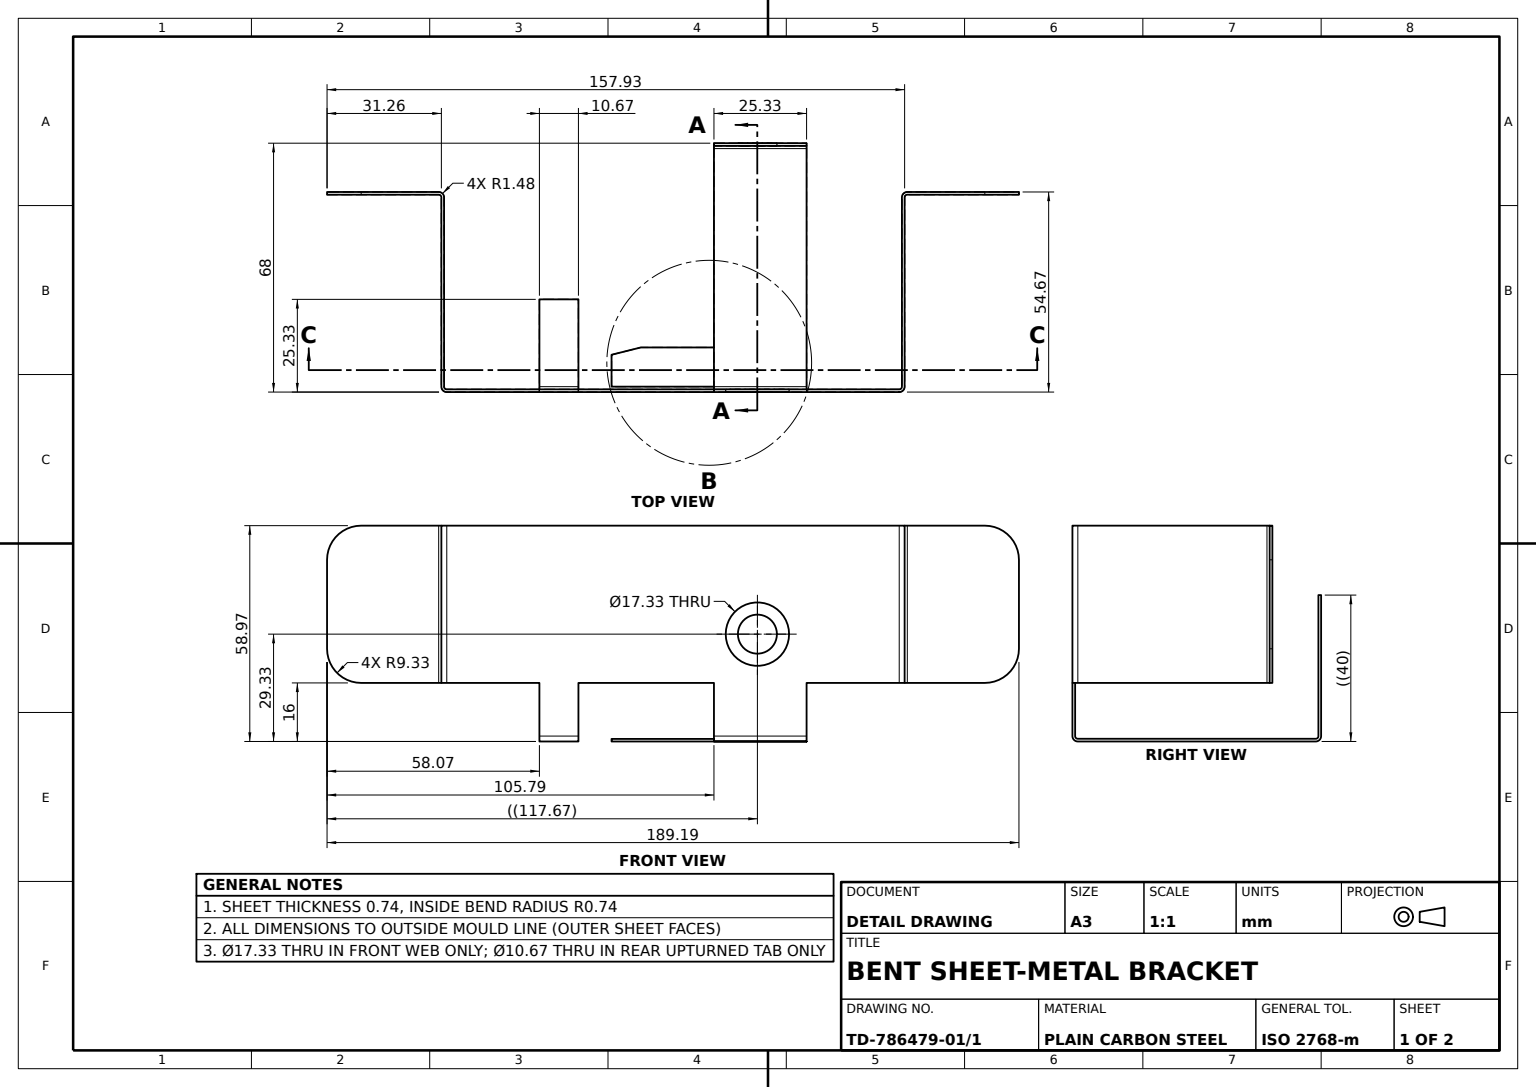
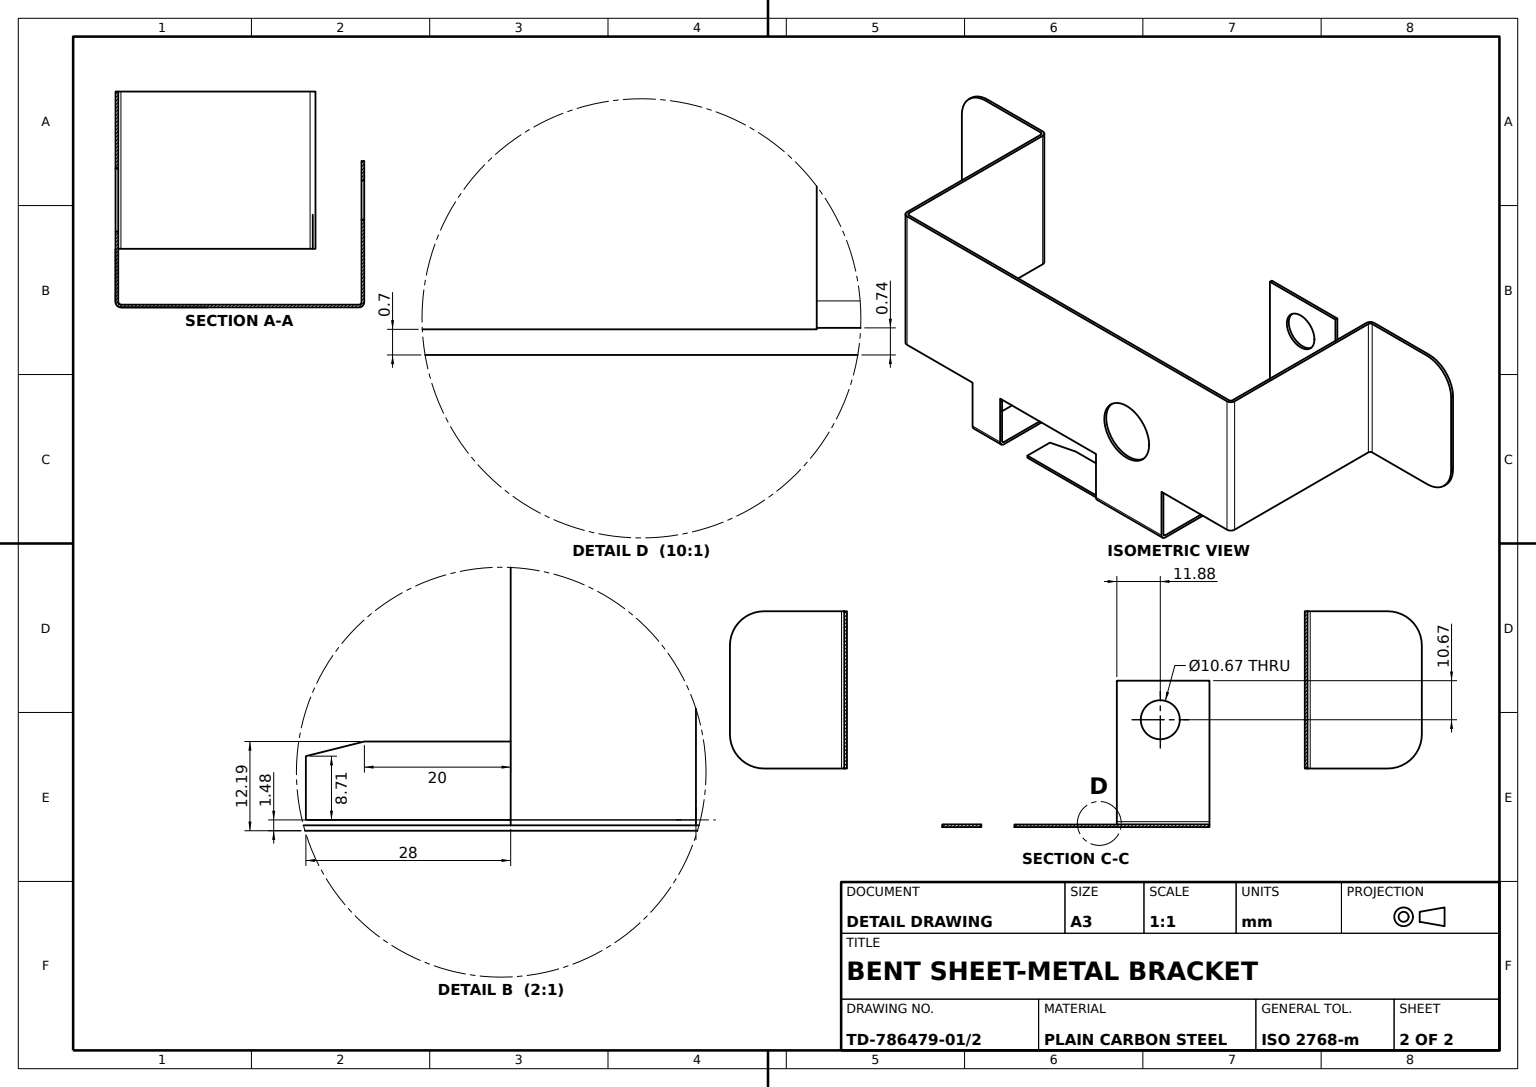
solid
v1 (11.1984,-36.745,-1.4766)
v2 (11.1984,-36.745,-66.5234)
e1 v1 v2 LINE
v3 (36.5284,-36.745,-1.4766)
e2 v3 v1 LINE
v4 (36.5284,-36.745,-66.5234)
e3 v4 v3 LINE
e4 v2 v4 LINE
face PLANE(AX(P(0,-36.745,0),D(0,1,0),D(0,0,1))) [-e1 -e2 -e3 -e4]
v5 (11.1984,-36.0084,0)
v6 (36.5284,-36.0084,0)
e5 v5 v6 LINE
v7 (11.1984,-37.485,-1.4766)
e6 v7 v5 CIRCLE(AX(P(11.1984,-36.0084,-1.4766),D(-1,0,0),D(0,0,1)),1.4766)
v8 (36.5284,-37.485,-1.4766)
e7 v7 v8 LINE
e8 v6 v8 CIRCLE(AX(P(36.5284,-36.0084,-1.4766),D(1,0,0),D(0,0,1)),1.4766)
face CYL(AX(P(11.1984,-36.0084,-1.4766),D(-1,0,0),D(0,-1,0)),1.4766) [-e5 -e6 e7 -e8]
v9 (-62.595,-21.485,-1.4766)
v10 (-63.335,-21.485,-1.4766)
e9 v9 v10 LINE
v11 (-61.8584,-21.485,-0.74)
e10 v11 v9 CIRCLE(AX(P(-61.8584,-21.485,-1.4766),D(0,-1,0),D(0,0,1)),0.7366)
v12 (-61.8584,-21.485,0)
e11 v11 v12 LINE
e12 v12 v10 CIRCLE(AX(P(-61.8584,-21.485,-1.4766),D(0,-1,0),D(0,0,1)),1.4766)
face PLANE(AX(P(-61.8584,-21.485,-1.4766),D(0,-1,0),D(0,0,-1))) [-e9 -e10 e11 e12]
v13 (-85.265,-21.485,-54.67)
v14 (-85.265,-21.485,-53.93)
e13 v13 v14 LINE
v15 (-94.595,-12.155,-53.93)
e14 v15 v14 CIRCLE(AX(P(-85.265,-12.155,-53.93),D(0,0,1),D(1,0,0)),9.33)
v16 (-94.595,-12.155,-54.67)
e15 v16 v15 LINE
e16 v16 v13 CIRCLE(AX(P(-85.265,-12.155,-54.67),D(0,0,1),D(1,0,0)),9.33)
face CYL(AX(P(-85.265,-12.155,-63.93),D(0,0,1),D(1,0,0)),9.33) [e13 -e14 -e15 e16]
v17 (85.265,-21.485,-54.67)
v18 (85.265,-21.485,-53.93)
e17 v17 v18 LINE
v19 (64.0716,-21.485,-53.93)
e18 v18 v19 LINE
v20 (64.0716,-21.485,-54.67)
e19 v19 v20 LINE
e20 v17 v20 LINE
face PLANE(AX(P(63.335,-21.485,-54.67),D(0,1,0),D(-1,0,0))) rev [e17 e18 e19 -e20]
v21 (11.1984,2.515,-68)
v22 (11.1984,2.515,-67.26)
e21 v21 v22 LINE
v23 (11.1984,-36.0084,-68)
e22 v23 v21 LINE
v24 (11.1984,-36.0084,-67.26)
e23 v24 v23 LINE
e24 v24 v22 LINE
face PLANE(AX(P(11.1984,2.515,-68),D(1,0,0),D(0,0,-1))) rev [-e21 -e22 -e23 e24]
v25 (-64.0716,-21.485,-54.67)
v26 (-64.0716,21.485,-54.67)
e25 v25 v26 LINE
v27 (-62.595,21.485,-53.1934)
e26 v27 v26 CIRCLE(AX(P(-64.0716,21.485,-53.1934),D(0,1,0),D(0,0,-1)),1.4766)
v28 (-62.595,-21.485,-53.1934)
e27 v28 v27 LINE
e28 v25 v28 CIRCLE(AX(P(-64.0716,-21.485,-53.1934),D(0,-1,0),D(0,0,-1)),1.4766)
face CYL(AX(P(-64.0716,-21.485,-53.1934),D(0,-1,0),D(0,0,-1)),1.4766) [e25 -e26 -e27 -e28]
v29 (36.5284,2.515,-67.26)
e29 v22 v29 LINE
v30 (36.5284,2.515,-68)
e30 v30 v29 LINE
e31 v21 v30 LINE
face PLANE(AX(P(36.5284,2.515,-68),D(0,-1,0),D(0,0,-1))) rev [e21 e29 -e30 -e31]
v31 (63.335,21.485,-53.1934)
v32 (62.595,21.485,-53.1934)
e32 v31 v32 LINE
v33 (62.595,21.485,-1.4766)
e33 v32 v33 LINE
v34 (63.335,21.485,-1.4766)
e34 v33 v34 LINE
e35 v31 v34 LINE
face PLANE(AX(P(63.335,21.485,-0.74),D(0,-1,0),D(1,0,0))) rev [e32 e33 e34 -e35]
v35 (-25.8584,-37.485,-25.33)
v36 (-25.8584,-36.745,-25.33)
e36 v35 v36 LINE
v37 (-25.8584,-36.745,-1.4766)
e37 v36 v37 LINE
v38 (-25.8584,-37.485,-1.4766)
e38 v37 v38 LINE
e39 v35 v38 LINE
face PLANE(AX(P(-25.8584,-37.485,-0.74),D(-1,0,0),D(0,0,1))) rev [e36 e37 e38 -e39]
v39 (-36.5284,-36.745,-25.33)
e40 v39 v36 LINE
v40 (-36.5284,-37.485,-25.33)
e41 v40 v35 LINE
e42 v40 v39 LINE
face PLANE(AX(P(-25.8584,-37.485,-25.33),D(0,0,1),D(0,-1,0))) rev [e40 -e36 -e41 e42]
v41 (36.5284,-21.485,0)
v42 (36.5284,-21.485,-0.74)
e43 v41 v42 LINE
e44 v6 v41 LINE
v43 (36.5284,-36.0084,-0.74)
e45 v43 v6 LINE
e46 v43 v42 LINE
face PLANE(AX(P(36.5284,-37.485,0),D(1,0,0),D(0,0,-1))) [-e43 -e44 -e45 e46]
v44 (-36.5284,-21.485,0)
e47 v12 v44 LINE
v45 (-36.5284,-36.0084,0)
e48 v45 v44 LINE
v46 (-25.8584,-36.0084,0)
e49 v45 v46 LINE
v47 (-25.8584,-21.485,0)
e50 v46 v47 LINE
v48 (11.1984,-21.485,0)
e51 v47 v48 LINE
e52 v5 v48 LINE
v49 (61.8584,-21.485,0)
e53 v41 v49 LINE
v50 (61.8584,21.485,0)
e54 v49 v50 LINE
v51 (-61.8584,21.485,0)
e55 v50 v51 LINE
e56 v51 v12 LINE
v52 (31.744549,-8.155,0)
v53 (14.414549,-8.155,0)
e57 v52 v53 CIRCLE(AX(P(23.079549,-8.155,0),D(0,0,-1),D(1,0,0)),8.665)
e58 v53 v52 CIRCLE(AX(P(23.079549,-8.155,0),D(0,0,-1),D(1,0,0)),8.665)
face PLANE(AX(P(36.5284,-37.485,0),D(0,0,-1),D(-1,0,0))) rev [e47 -e48 e49 e50 e51 -e52 e5 e44 e53 e54 e55 e56] [e57 e58]
v54 (61.8584,21.485,-0.74)
v55 (-61.8584,21.485,-0.74)
e59 v54 v55 LINE
e60 v55 v51 LINE
e61 v54 v50 LINE
face PLANE(AX(P(-63.335,21.485,-0.74),D(0,1,0),D(0,0,1))) [e59 e60 -e55 -e61]
e62 v25 v13 LINE
v56 (-64.0716,-21.485,-53.93)
e63 v56 v25 LINE
e64 v56 v14 LINE
face PLANE(AX(P(-94.595,-21.485,-54.67),D(0,1,0),D(0,0,1))) rev [-e62 -e63 e64 -e13]
e65 v3 v8 LINE
v57 (36.5284,-37.485,-66.5234)
e66 v57 v8 LINE
e67 v4 v57 LINE
face PLANE(AX(P(36.5284,-37.485,-0.74),D(-1,0,0),D(0,-1,0))) rev [e3 e65 -e66 -e67]
v58 (-36.5284,-21.485,-0.74)
e68 v58 v44 LINE
v59 (-36.5284,-36.0084,-0.74)
e69 v59 v58 LINE
e70 v59 v45 LINE
face PLANE(AX(P(-36.5284,-37.485,0),D(-1,0,0),D(0,0,1))) [e48 -e68 -e69 e70]
v60 (11.1984,-36.0084,-0.74)
e71 v60 v5 LINE
e72 v1 v60 CIRCLE(AX(P(11.1984,-36.0084,-1.4766),D(-1,0,0),D(0,0,1)),0.7366)
e73 v1 v7 LINE
face PLANE(AX(P(11.1984,-36.0084,-1.4766),D(1,0,0),D(0,0,-1))) rev [-e71 -e72 e73 e6]
v61 (94.595,12.155,-53.93)
v62 (94.595,-12.155,-53.93)
e74 v61 v62 LINE
v63 (94.595,-12.155,-54.67)
e75 v62 v63 LINE
v64 (94.595,12.155,-54.67)
e76 v64 v63 LINE
e77 v61 v64 LINE
face PLANE(AX(P(94.595,-21.485,-54.67),D(-1,0,0),D(0,-1,0))) rev [e74 e75 -e76 -e77]
e78 v63 v17 CIRCLE(AX(P(85.265,-12.155,-54.67),D(0,0,-1),D(1,0,0)),9.33)
v65 (64.0716,21.485,-54.67)
e79 v65 v20 LINE
v66 (85.265,21.485,-54.67)
e80 v65 v66 LINE
e81 v66 v64 CIRCLE(AX(P(85.265,12.155,-54.67),D(0,0,-1),D(1,0,0)),9.33)
face PLANE(AX(P(0,0,-54.67),D(0,0,1),D(1,0,0))) rev [e78 e20 -e79 e80 e81 e76]
v67 (-36.5284,-36.745,-1.4766)
e82 v37 v67 LINE
e83 v67 v59 CIRCLE(AX(P(-36.5284,-36.0084,-1.4766),D(-1,0,0),D(0,0,1)),0.7366)
v68 (-25.8584,-36.0084,-0.74)
e84 v59 v68 LINE
e85 v68 v37 CIRCLE(AX(P(-25.8584,-36.0084,-1.4766),D(1,0,0),D(0,0,1)),0.7366)
face CYL(AX(P(-36.5284,-36.0084,-1.4766),D(-1,0,0),D(0,-1,0)),0.7366) rev [e82 e83 e84 e85]
e86 v62 v18 CIRCLE(AX(P(85.265,-12.155,-53.93),D(0,0,-1),D(1,0,0)),9.33)
face CYL(AX(P(85.265,-12.155,-63.93),D(0,0,1),D(1,0,0)),9.33) [-e17 -e78 -e75 e86]
e87 v65 v32 CIRCLE(AX(P(64.0716,21.485,-53.1934),D(0,1,0),D(0,0,1)),1.4766)
v69 (62.595,-21.485,-53.1934)
e88 v69 v20 CIRCLE(AX(P(64.0716,-21.485,-53.1934),D(0,-1,0),D(0,0,1)),1.4766)
e89 v32 v69 LINE
face CYL(AX(P(64.0716,21.485,-53.1934),D(0,1,0),D(0,0,-1)),1.4766) [-e87 e79 -e88 -e89]
v70 (14.414549,-8.155,-0.74)
e90 v70 v53 LINE
v71 (31.744549,-8.155,-0.74)
e91 v71 v52 LINE
e92 v71 v70 CIRCLE(AX(P(23.079549,-8.155,-0.74),D(0,0,-1),D(1,0,0)),8.665)
face CYL(AX(P(23.079549,-8.155,-33.74),D(0,0,1),D(1,0,0)),8.665) rev [e90 -e57 -e91 e92]
v72 (62.595,-21.485,-1.4766)
e93 v72 v69 LINE
v73 (63.335,-21.485,-53.1934)
e94 v73 v69 LINE
v74 (63.335,-21.485,-1.4766)
e95 v74 v73 LINE
e96 v72 v74 LINE
face PLANE(AX(P(63.335,-21.485,-54.67),D(0,1,0),D(-1,0,0))) rev [e93 -e94 -e95 -e96]
v75 (61.8584,-21.485,-0.74)
e97 v75 v49 LINE
e98 v72 v75 CIRCLE(AX(P(61.8584,-21.485,-1.4766),D(0,-1,0),D(0,0,-1)),0.7366)
e99 v74 v49 CIRCLE(AX(P(61.8584,-21.485,-1.4766),D(0,-1,0),D(0,0,-1)),1.4766)
face PLANE(AX(P(61.8584,-21.485,-1.4766),D(0,1,0),D(0,0,1))) rev [-e97 -e98 e96 e99]
e100 v43 v3 CIRCLE(AX(P(36.5284,-36.0084,-1.4766),D(1,0,0),D(0,0,1)),0.7366)
face PLANE(AX(P(36.5284,-36.0084,-1.4766),D(1,0,0),D(0,0,-1))) [-e100 e45 e8 -e65]
v76 (17.744549,-8.155,-68)
v77 (17.744549,-8.155,-67.26)
e101 v76 v77 LINE
v78 (28.414549,-8.155,-68)
e102 v76 v78 CIRCLE(AX(P(23.079549,-8.155,-68),D(0,0,-1),D(0,-1,0)),5.335)
v79 (28.414549,-8.155,-67.26)
e103 v78 v79 LINE
e104 v77 v79 CIRCLE(AX(P(23.079549,-8.155,-67.26),D(0,0,-1),D(0,-1,0)),5.335)
face CYL(AX(P(23.079549,-8.155,-73.74),D(0,0,1),D(1,0,0)),5.335) rev [-e101 e102 e103 -e104]
v80 (64.0716,21.485,-53.93)
v81 (85.265,21.485,-53.93)
e105 v80 v81 LINE
e106 v66 v81 LINE
e107 v80 v65 LINE
face PLANE(AX(P(94.595,21.485,-54.67),D(0,-1,0),D(1,0,0))) rev [e105 -e106 -e80 -e107]
e108 v68 v46 LINE
e109 v46 v38 CIRCLE(AX(P(-25.8584,-36.0084,-1.4766),D(1,0,0),D(0,0,1)),1.4766)
face PLANE(AX(P(-25.8584,-36.0084,-1.4766),D(1,0,0),D(0,0,-1))) [-e38 -e85 e108 e109]
v82 (-85.265,21.485,-54.67)
v83 (-94.595,12.155,-54.67)
e110 v82 v83 CIRCLE(AX(P(-85.265,12.155,-54.67),D(0,0,1),D(1,0,0)),9.33)
e111 v82 v26 LINE
e112 v16 v83 LINE
face PLANE(AX(P(0,0,-54.67),D(0,0,1),D(1,0,0))) rev [-e110 e111 -e25 e62 -e16 e112]
v84 (-63.335,21.485,-1.4766)
e113 v84 v10 LINE
v85 (-63.335,21.485,-53.1934)
e114 v84 v85 LINE
v86 (-63.335,-21.485,-53.1934)
e115 v86 v85 LINE
e116 v86 v10 LINE
face PLANE(AX(P(-63.335,0,0),D(1,0,0),D(0,0,-1))) rev [-e113 e114 -e115 e116]
v87 (-94.595,12.155,-53.93)
e117 v15 v87 LINE
e118 v83 v87 LINE
face PLANE(AX(P(-94.595,21.485,-54.67),D(1,0,0),D(0,0,-1))) rev [e117 -e118 -e112 e15]
v88 (-8.8016,-36.785,-12.19)
v89 (11.1984,-36.785,-12.19)
e119 v88 v89 LINE
v90 (11.1984,-37.485,-12.19)
e120 v89 v90 LINE
v91 (-8.8016,-37.485,-12.19)
e121 v91 v90 LINE
e122 v88 v91 LINE
face PLANE(AX(P(11.1984,-36.785,-12.19),D(0,0,-1),D(0,1,0))) [e119 e120 -e121 -e122]
e123 v67 v39 LINE
face PLANE(AX(P(0,-36.745,0),D(0,1,0),D(0,0,1))) [-e37 -e40 -e123 -e82]
e124 v60 v43 LINE
face CYL(AX(P(11.1984,-36.0084,-1.4766),D(-1,0,0),D(0,-1,0)),0.7366) rev [e124 e100 e2 e72]
v92 (-62.595,21.485,-1.4766)
e125 v92 v27 LINE
e126 v9 v92 LINE
e127 v28 v9 LINE
face PLANE(AX(P(-62.595,0,0),D(1,0,0),D(0,0,-1))) [-e125 -e126 -e127 e27]
e128 v70 v71 CIRCLE(AX(P(23.079549,-8.155,-0.74),D(0,0,-1),D(1,0,0)),8.665)
face CYL(AX(P(23.079549,-8.155,-33.74),D(0,0,1),D(1,0,0)),8.665) rev [e91 -e58 -e90 e128]
e129 v92 v55 CIRCLE(AX(P(-61.8584,21.485,-1.4766),D(0,1,0),D(0,0,1)),0.7366)
e130 v55 v11 LINE
face CYL(AX(P(-61.8584,21.485,-1.4766),D(0,1,0),D(-1,0,0)),0.7366) rev [e129 e130 e10 e126]
v93 (-25.8584,-21.485,-0.74)
e131 v93 v47 LINE
e132 v68 v93 LINE
face PLANE(AX(P(-25.8584,-37.485,0),D(-1,0,0),D(0,0,1))) rev [e131 -e50 -e108 e132]
e133 v86 v28 LINE
e134 v56 v86 CIRCLE(AX(P(-64.0716,-21.485,-53.1934),D(0,-1,0),D(0,0,-1)),0.7366)
face PLANE(AX(P(-64.0716,-21.485,-53.1934),D(0,1,0),D(0,0,1))) rev [-e133 -e134 e63 e28]
v94 (-64.0716,21.485,-53.93)
e135 v94 v26 LINE
e136 v85 v94 CIRCLE(AX(P(-64.0716,21.485,-53.1934),D(0,1,0),D(0,0,-1)),0.7366)
e137 v85 v27 LINE
face PLANE(AX(P(-64.0716,21.485,-53.1934),D(0,1,0),D(0,0,1))) [e26 -e135 -e136 e137]
e138 v80 v31 CIRCLE(AX(P(64.0716,21.485,-53.1934),D(0,1,0),D(0,0,1)),0.7366)
face PLANE(AX(P(64.0716,21.485,-53.1934),D(0,-1,0),D(0,0,-1))) rev [-e32 -e138 e107 e87]
v95 (11.1984,-37.485,-1.48)
v96 (-16.8016,-37.485,-1.48)
e139 v95 v96 LINE
v97 (11.1984,-36.785,-1.48)
e140 v97 v95 LINE
v98 (-16.8016,-36.785,-1.48)
e141 v97 v98 LINE
e142 v98 v96 LINE
face PLANE(AX(P(11.1984,-36.785,-1.48),D(0,0,1),D(0,-1,0))) [-e139 -e140 e141 e142]
e143 v74 v34 LINE
e144 v50 v34 CIRCLE(AX(P(61.8584,21.485,-1.4766),D(0,1,0),D(0,0,-1)),1.4766)
face CYL(AX(P(61.8584,-21.485,-1.4766),D(0,-1,0),D(1,0,0)),1.4766) [-e54 -e99 e143 -e144]
e145 v81 v61 CIRCLE(AX(P(85.265,12.155,-53.93),D(0,0,-1),D(1,0,0)),9.33)
face CYL(AX(P(85.265,12.155,-63.93),D(0,0,1),D(1,0,0)),9.33) [e106 e145 e77 -e81]
v99 (11.1984,-37.485,-66.5234)
e146 v90 v99 LINE
e147 v89 v97 LINE
e148 v7 v95 LINE
e149 v2 v99 LINE
face PLANE(AX(P(11.1984,-37.485,-68),D(1,0,0),D(0,1,0))) rev [-e146 -e120 e147 e140 -e148 -e73 e1 e149]
v100 (-36.5284,-37.485,-1.4766)
e150 v100 v45 CIRCLE(AX(P(-36.5284,-36.0084,-1.4766),D(-1,0,0),D(0,0,1)),1.4766)
e151 v100 v38 LINE
face CYL(AX(P(-36.5284,-36.0084,-1.4766),D(-1,0,0),D(0,-1,0)),1.4766) [-e109 -e49 -e150 e151]
v101 (36.5284,-36.0084,-67.26)
e152 v4 v101 CIRCLE(AX(P(36.5284,-36.0084,-66.5234),D(1,0,0),D(0,0,1)),0.7366)
e153 v101 v24 LINE
e154 v24 v2 CIRCLE(AX(P(11.1984,-36.0084,-66.5234),D(-1,0,0),D(0,0,1)),0.7366)
face CYL(AX(P(11.1984,-36.0084,-66.5234),D(-1,0,0),D(0,0,-1)),0.7366) rev [e152 e153 e154 e4]
e155 v23 v99 CIRCLE(AX(P(11.1984,-36.0084,-66.5234),D(-1,0,0),D(0,0,1)),1.4766)
face PLANE(AX(P(11.1984,-36.0084,-66.5234),D(1,0,0),D(0,0,-1))) rev [-e149 -e154 e23 e155]
e156 v19 v80 LINE
face PLANE(AX(P(0,0,-53.93),D(0,0,1),D(1,0,0))) [-e105 -e156 -e18 -e86 -e74 -e145]
e157 v75 v54 LINE
e158 v42 v75 LINE
v102 (11.1984,-21.485,-0.74)
e159 v60 v102 LINE
e160 v93 v102 LINE
e161 v11 v58 LINE
face PLANE(AX(P(36.5284,-37.485,-0.74),D(0,0,-1),D(-1,0,0))) [-e59 -e157 -e158 -e46 -e124 e159 -e160 -e132 -e84 e69 -e161 -e130] [-e92 -e128]
face PLANE(AX(P(-63.335,-21.485,-0.74),D(0,-1,0),D(0,0,-1))) [-e11 e161 e68 -e47]
v103 (-16.8016,-37.485,-10.19)
e162 v96 v103 LINE
v104 (-16.8016,-36.785,-10.19)
e163 v98 v104 LINE
e164 v104 v103 LINE
face PLANE(AX(P(-16.8016,-36.785,-1.48),D(-1,0,0),D(0,-1,0))) [-e162 -e142 e163 e164]
e165 v102 v48 LINE
face PLANE(AX(P(11.1984,-37.485,-0.74),D(-1,0,0),D(0,0,1))) [e71 e52 -e165 -e159]
v105 (36.5284,-36.0084,-68)
e166 v23 v105 LINE
e167 v57 v105 CIRCLE(AX(P(36.5284,-36.0084,-66.5234),D(1,0,0),D(0,0,1)),1.4766)
e168 v99 v57 LINE
face CYL(AX(P(11.1984,-36.0084,-66.5234),D(-1,0,0),D(0,0,-1)),1.4766) [e166 -e167 -e168 -e155]
v106 (-85.265,21.485,-53.93)
e169 v106 v87 CIRCLE(AX(P(-85.265,12.155,-53.93),D(0,0,1),D(1,0,0)),9.33)
e170 v82 v106 LINE
face CYL(AX(P(-85.265,12.155,-63.93),D(0,0,1),D(1,0,0)),9.33) [-e169 -e170 e110 e118]
e171 v104 v88 LINE
e172 v103 v91 LINE
face PLANE(AX(P(-8.8016,-36.785,-12.19),D(-0.242535625,0,-0.9701425),D(-0.9701425,0,0.242535625))) [-e164 e171 e122 -e172]
e173 v54 v33 CIRCLE(AX(P(61.8584,21.485,-1.4766),D(0,1,0),D(0,0,-1)),0.7366)
face PLANE(AX(P(61.8584,21.485,-1.4766),D(0,1,0),D(0,0,1))) [-e34 -e173 e61 e144]
e174 v92 v84 LINE
e175 v84 v51 CIRCLE(AX(P(-61.8584,21.485,-1.4766),D(0,1,0),D(0,0,1)),1.4766)
face PLANE(AX(P(-61.8584,21.485,-1.4766),D(0,-1,0),D(0,0,-1))) rev [e174 e175 -e60 -e129]
e176 v33 v72 LINE
face CYL(AX(P(61.8584,-21.485,-1.4766),D(0,-1,0),D(1,0,0)),0.7366) rev [e176 e98 e157 e173]
e177 v94 v56 LINE
face CYL(AX(P(-64.0716,-21.485,-53.1934),D(0,-1,0),D(0,0,-1)),0.7366) rev [e177 e134 e115 e136]
e178 v101 v105 LINE
face PLANE(AX(P(36.5284,-36.0084,-66.5234),D(1,0,0),D(0,0,-1))) [-e178 -e152 e67 e167]
e179 v67 v100 LINE
face PLANE(AX(P(-36.5284,-36.0084,-1.4766),D(1,0,0),D(0,0,-1))) rev [-e70 -e83 e179 e150]
e180 v78 v76 CIRCLE(AX(P(23.079549,-8.155,-68),D(0,0,-1),D(0,-1,0)),5.335)
e181 v79 v77 CIRCLE(AX(P(23.079549,-8.155,-67.26),D(0,0,-1),D(0,-1,0)),5.335)
face CYL(AX(P(23.079549,-8.155,-73.74),D(0,0,1),D(1,0,0)),5.335) rev [e180 e101 -e181 -e103]
e182 v29 v101 LINE
e183 v30 v105 LINE
face PLANE(AX(P(36.5284,-36.745,-68),D(-1,0,0),D(0,0,1))) rev [e30 e182 e178 -e183]
face PLANE(AX(P(-63.335,-21.485,-0.74),D(0,-1,0),D(0,0,-1))) [e165 -e51 -e131 e160]
e184 v106 v94 LINE
face PLANE(AX(P(-63.335,21.485,-54.67),D(0,-1,0),D(0,0,-1))) rev [e135 -e111 e170 e184]
e185 v100 v40 LINE
face PLANE(AX(P(0,-37.485,0),D(0,1,0),D(0,0,1))) rev [e39 -e151 e185 e41]
e186 v73 v19 CIRCLE(AX(P(64.0716,-21.485,-53.1934),D(0,-1,0),D(0,0,1)),0.7366)
face PLANE(AX(P(64.0716,-21.485,-53.1934),D(0,-1,0),D(0,0,-1))) [-e19 -e186 e94 e88]
face PLANE(AX(P(0,-37.485,0),D(0,1,0),D(0,0,1))) rev [e172 e121 e146 e168 e66 -e7 e148 e139 e162]
face PLANE(AX(P(-63.335,21.485,-54.67),D(0,-1,0),D(0,0,-1))) rev [-e114 -e174 e125 -e137]
e187 v31 v73 LINE
face CYL(AX(P(64.0716,21.485,-53.1934),D(0,1,0),D(0,0,-1)),0.7366) rev [e186 e156 e138 e187]
face PLANE(AX(P(63.335,0,0),D(-1,0,0),D(0,0,1))) rev [-e143 e95 -e187 e35]
face PLANE(AX(P(-36.5284,-37.485,-25.33),D(1,0,0),D(0,0,-1))) rev [-e185 -e179 e123 -e42]
face PLANE(AX(P(0,0,-53.93),D(0,0,1),D(1,0,0))) [e169 -e117 e14 -e64 -e177 -e184]
face PLANE(AX(P(0,0,-68),D(0,0,1),D(0,-1,0))) rev [-e180 -e102] [e31 e183 -e166 e22]
face PLANE(AX(P(0,0,-67.26),D(0,0,1),D(0,-1,0))) [e181 e104] [-e29 -e24 -e153 -e182]
face CYL(AX(P(-61.8584,21.485,-1.4766),D(0,1,0),D(-1,0,0)),1.4766) [-e12 -e56 -e175 e113]
face PLANE(AX(P(-63.335,-21.485,-0.74),D(0,1,0),D(0,0,1))) rev [e133 e127 e9 -e116]
face PLANE(AX(P(0,-36.785,0),D(0,1,0),D(0,0,1))) [-e119 -e171 -e163 -e141 -e147]
face PLANE(AX(P(-63.335,-21.485,-0.74),D(0,-1,0),D(0,0,-1))) [e43 e158 e97 -e53]
face PLANE(AX(P(62.595,0,0),D(-1,0,0),D(0,0,1))) [-e176 -e33 e89 -e93]
